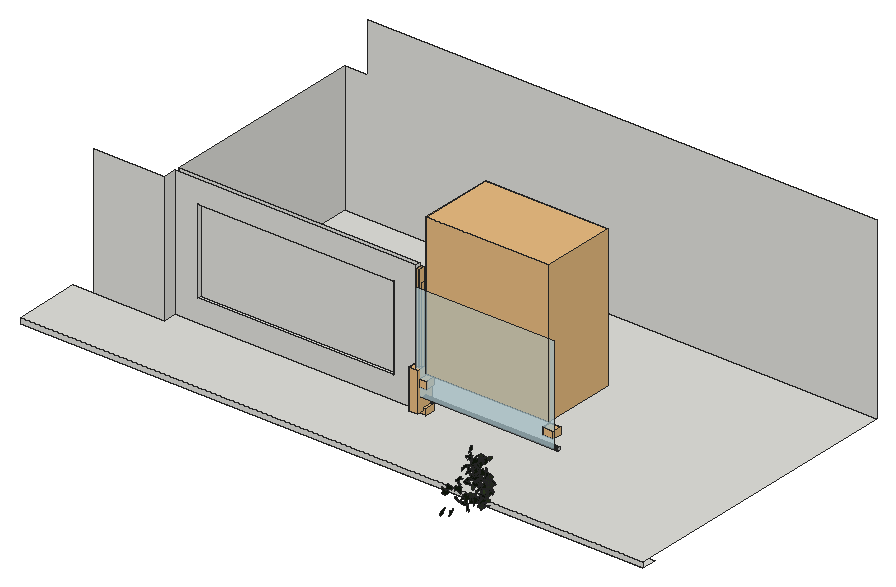
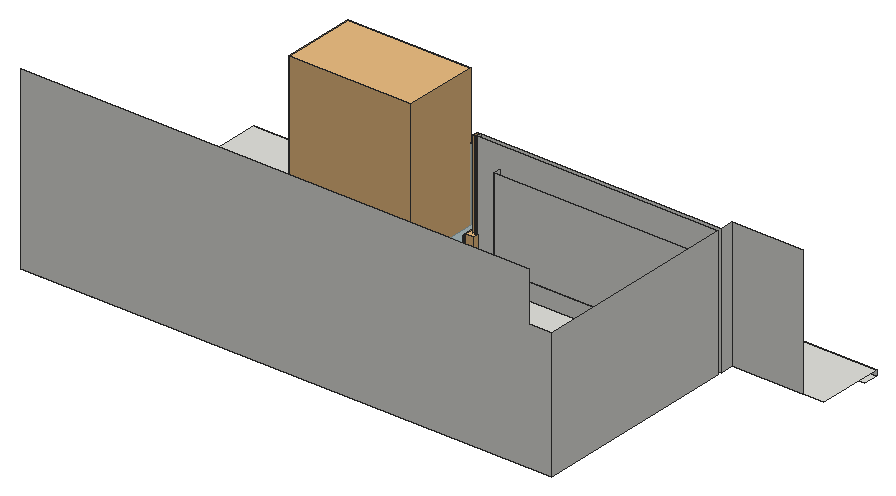
# SketchUp Ruby script. Lengths in inches.
U = 1.inch
M = Sketchup.active_model
def pt(a) = Geom::Point3d.new(a.map { |v| v * U })
def face(e, loops, mat)
  f = e.add_face(loops[0].map { |a| pt(a) })
  loops[1..].each { |l| e.add_face(l.map { |a| pt(a) }).erase! }
  f.material = f.back_material = mat if mat
  f
end
# faces: each face lists its corners as indices into pts; further lists are holes
def faces(e, pts, list, mat = nil) = list.each { |f| face(e, (f[0].is_a?(Array) ? f : [f]).map { |l| l.map { |i| pts[i] } }, mat) }
# xy, xz, yz: faces in a plane at the given z, y or x. An outline is a flat list of corners, or four numbers for a rectangle; further outlines are holes
def ring(l) = l.size == 4 ? [[l[0], l[1]], [l[2], l[1]], [l[2], l[3]], [l[0], l[3]]] : l.each_slice(2).to_a
def flat(e, list, mat, &to3) = list.each { |f| face(e, (f[0].is_a?(Array) ? f : [f]).map { |l| ring(l).map { |u, v| to3.(u, v) } }, mat) }
def xy(e, z, list, mat = nil) = flat(e, list, mat) { |x, y| [x, y, z] }
def xz(e, y, list, mat = nil) = flat(e, list, mat) { |x, z| [x, y, z] }
def yz(e, x, list, mat = nil) = flat(e, list, mat) { |y, z| [x, y, z] }
def lines(e, pts, list) = list.each { |a, b| e.add_line(pt(pts[a]), pt(pts[b])) }
# prism: a flat outline (further loops are holes) pulled along v
def prism(e, loops, v, mat = nil)
  f = face(e, loops, mat); d = Geom::Vector3d.new(v.map { |x| x * U })
  f.pushpull(f.normal.samedirection?(d) ? d.length : -d.length)
end
def box(e, o, s, mat = nil) = prism(e, [[o, [o[0] + s[0], o[1], o[2]], [o[0] + s[0], o[1] + s[1], o[2]], [o[0], o[1] + s[1], o[2]]]], [0, 0, s[2]], mat)
def at(x, y, z, deg = 0) = Geom::Transformation.translation(pt([x, y, z])) * Geom::Transformation.rotation(ORIGIN, Z_AXIS, deg.degrees)
def axes(o, x, y, z) = Geom::Transformation.new([*x, 0, *y, 0, *z, 0, *pt(o).to_a, 1])
def part(name) = M.definitions.add(name)
# library, detail: a bought-in or finely detailed component or shape, given as its bounding box
def library(name, o, s) = part(name).tap { |d| box(d.entities, o, s) }
def detail(e, o, s) = box(e.add_group.entities, o, s)
def put(e, d, t, mat = nil) = e.add_instance(d, t).tap { |i| i.material = mat if mat }
def group(e, t, mat = nil) = e.add_group.tap { |g| g.transformation = t; g.material = mat if mat }.entities
root = M.entities
M.materials.add("Glass Rail Metal").color = [192, 192, 192]
M.materials.add("[Translucent Glass Safety]").color = [204, 235, 244]
M.materials["[Translucent Glass Safety]"].alpha = 0.5
M.materials.add("[Translucent Glass Tinted]").color = [8, 201, 241]
M.materials["[Translucent Glass Tinted]"].alpha = 0.48
M.materials.add("efeu1").color = [18, 25, 13]
M.materials.add("efeu2").color = [43, 57, 29]
c1 = library("Group\#37",[0,0,0],[3.67,3.3,2.01])
c2 = library("Group\#43",[0,0,0],[50.8,6,878.92])
c3 = library("Group\#53",[0,0,0],[3.15,5.91,11.14])
c4 = library("Group\#15",[0.69,0,0.79],[0.62,1.89,30.3])
c5 = library("Group\#46",[0,0,0],[50.8,6,878.92])
c6 = library("glass bracket3",[-2.83,-0.98,-1],[3.67,3.29,2])
c7 = library("Palm+in+pot",[-44.1,-44.03,0.04],[106.77,95.72,88.04])
c8 = part("ivyleaf_9")
p = [[1.54,2.16,1.25],[1.36,2.04,1.19],[-0.21,0.99,0.68],[-0.71,1.11,0.82],[-0.85,0.86,0.67],[-0.8,0.17,0.21],
  [-0.9,-0.01,0.1],[-0.67,-0.16,-0.02],[-0.08,-0.08,-0.05],[-0.03,-0.6,-0.4],[0.65,-0.88,-0.66],[0.83,-0.6,-0.49],
  [1.29,-0.42,-0.43],[1.8125,-0.07,-0.26],[1.21,0.44,0.15]]
faces(c8.entities,p,[[0,1,2,3,4,5,6,7,8,9,10,11,12,13,14]],"efeu1")
c9 = part("ivyleaf_10")
p = [[0,0.5,-0.03],[-0.0625,2.02,-0.43],[-0.19,2.01,-0.46],[-0.54,1.05,-0.29],[-0.52,0.625,-0.18],[-0.83,0.76,-0.28],
  [-1.16,0.64,-0.33],[-1.15,0.33,-0.24],[-0.77,-0.39,0.02],[-0.3,-0.51,0.16],[0.04,-0.48,0.23],[-0.02,2.01,-0.4375],
  [-0.06,2.01,-0.43],[0.04,-0.49,0.23],[0.67,-0.49,0.14],[1.38,0.36,-0.2],[1.375,0.51,-0.24],[0.81,0.65,-0.19],
  [0.62,0.59,-0.15],[0.6,1.09,-0.28],[0.5,1.23,-0.31]]
faces(c9.entities,p,[[0,1,2,3,4,5,6,7,8,9,10],[11,12,0,13,14,15,16,17,18,19,20]],"efeu2")
c10 = library("glass bracket3\#1",[-0.84,-0.98,-1],[3.67,3.29,2])
prism(root,[[[415.35,181.67,254.4375],[415.35,181.84,254.35],[415.35,181.98,254.2],[415.35,182.09,254.02],[415.35,182.16,253.8125],[415.35,182.17,253.59],[415.35,182.14,253.375],[415.35,182.0625,253.18],[415.35,181.94,253.01],[415.35,181.79,252.88],[415.35,181.61,252.8],[415.35,181.43,252.78],[415.35,181.25,252.82],[415.35,181.08,252.91],[415.35,180.93,253.06],[415.35,180.83,253.24],[415.35,180.76,253.45],[415.35,180.75,253.67],[415.35,180.78,253.88],[415.35,180.86,254.09],[415.35,180.98,254.26],[415.35,181.13,254.38],[415.35,181.3,254.46],[415.35,181.49,254.48]]],[89.11,0,0],"Glass Rail Metal")
box(root,[415.02,177.2,254.7],[89.77,0.59,63.38],"[Translucent Glass Safety]")
xy(root,240.74,[[196.34,130,600,139.625]])
xy(root,244.35,[[196.34,130,600,130,600,319,255.63,319,255.63,184.12,411.76,184.12,411.76,181.4375,255.63,181.4375,255.63,172.6875,196.34,172.6875]])
xy(root,258.8125,[[270.09,181.4375,397.3,188.5625]])
xz(root,130,[[196.34,240.74,600,244.35]])
xz(root,172.6875,[[209.625,244.35,255.63,328.1875]])
xz(root,181.4375,[[[255.63,244.35,411.76,328.1875],[270.09,258.8125,397.3,313.73]]])
xz(root,184.12,[[255.63,244.35,411.76,328.1875]])
xz(root,188.5625,[[270.09,258.8125,397.3,313.73]])
xz(root,319,[[255.63,244.35,600,244.35,600,360,270.19,360,270.19,328.1875,255.63,328.1875]])
yz(root,255.63,[[172.6875,244.35,181.4375,328.1875],[184.12,244.35,319,328.1875]])
yz(root,270.09,[[181.4375,258.8125,188.5625,313.73]])
yz(root,397.3,[[181.4375,258.8125,188.5625,313.73]])
yz(root,411.76,[[181.4375,244.35,184.12,328.1875]])
put(root,c1,axes([408.92,179.59,243.35],[1.9,0,0],[0,1.9,0],[0,0,2.261]),"[Translucent Glass Tinted]")
put(root,c2,axes([413.71,179.56,248.78],[0,0.0748,0],[-0.0748,0,0.00001],[0.00001,0,0.08902]),"[Translucent Glass Tinted]")
put(root,c3,axes([411.3125,175.85,245.62],[1.9,0,0],[0,1.9,0],[0,0,2.261]),"[Translucent Glass Tinted]")
put(root,c4,axes([416.1,179.56,248.78],[0,1.9,0],[-1.9,0,0.00031],[0.00026,0,2.261]),"Glass Rail Metal")
put(root,c5,axes([415.35,179.56,248.78],[0,0.0748,0],[-0.0748,0,0.00001],[0.00001,0,0.08902]),"[Translucent Glass Tinted]")
put(root,c1,axes([419.68,179.59,247.89],[-1.9,0,0.00031],[0,1.9,0],[-0.00026,0,-2.261]),"[Translucent Glass Tinted]")
put(root,c6,axes([420.75,178.46,263.5625],[1.9,0,0],[0,1.9,0],[0,0,2.261]),"[Translucent Glass Tinted]")
put(root,c7,axes([454.51,199.21,269.81],[0.74365,0,0],[0,0.5,0],[0,0,1.0374]))
put(root,c8,axes([489.26,108.62,254.52],[0.59442,0.04762,1.18171],[-1.2151,0.20696,0.55776],[-0.17918,-1.24547,0.13787]))
put(root,c8,axes([489.92,123.09,263.95],[-0.23632,0.9466,-0.70763],[0.0907,-0.6777,-1.00862],[-1.25576,-0.22709,0.06031]))
put(root,c8,axes([489.8,104.18,244.44],[-0.48717,1.15827,0.44196],[0.13676,-0.40662,1.2924],[1.32543,0.46768,0.02909]))
put(root,c8,axes([490.71,109.53,258.73],[0.46963,0.40029,-1.13624],[-0.84856,-0.75927,-0.61453],[-0.92689,0.89792,-0.01311]))
put(root,c8,axes([491.32,124.37,256.75],[-0.12929,0.9505,-0.65584],[0.06165,-0.6283,-0.99615],[-1.23038,-0.13136,0.01901]))
put(root,c8,axes([492.43,109.09,243.9],[-0.46395,0.88248,0.8737],[-0.38333,0.7615,-1.02068],[-1.25881,-0.55714,-0.01119]))
put(root,c8,axes([492.08,114.92,260.75],[0.50243,0.7718,0.79926],[0.44241,0.65035,-0.93714],[-1.08994,0.61975,-0.01195]))
put(root,c8,axes([492.99,125.8125,244.46],[-1.16401,0.10836,-0.03835],[0.03948,-0.00498,-1.12655],[-0.11714,-1.07841,0.00135]))
put(root,c8,axes([492.79,122.28,264.03],[0.70443,-0.28766,-0.9331],[-0.88039,0.3749,-0.74133],[0.51027,1.04397,0.00911]))
put(root,c8,axes([492.25,114.53,256.4375],[-0.32312,-0.76804,-0.94362],[0.3738,0.83881,-0.85714],[1.22823,-0.45734,0.01261]))
put(root,c8,axes([491.68,114.18,249.6],[0.81283,-0.58166,0.82454],[0.66536,-0.49923,-0.98913],[0.82771,0.97252,-0.0146]))
put(root,c8,axes([492.22,114.51,259.49],[1.15165,-0.29641,-0.49126],[0.5136,-0.04902,1.14849],[-0.31455,-1.16525,0.07665]))
put(root,c8,axes([493.375,124.24,275.64],[-0.96606,0.3245,-0.62908],[0.60337,-0.23314,-0.98928],[-0.43074,-1.05435,0.02514]))
put(root,c8,axes([492.61,118.95,245.04],[1.18089,0.48616,0.00947],[-0.01579,0.01049,1.24438],[0.52491,-1.0934,0.01615]))
put(root,c9,axes([494.01,124.91,251.71],[-0.01496,0.96068,-0.5547],[-0.26695,0.51701,0.97515],[1.1563,0.13179,0.21795]))
put(root,c9,axes([493.64,126.24,247.0625],[1.13658,0.27915,-0.10532],[-0.09971,-0.04684,-1.13211],[-0.30482,1.05621,-0.02237]))
put(root,c8,axes([494.28,118.25,250.64],[-0.20997,0.14185,-1.19782],[0.28117,-1.1327,-0.19079],[-1.22134,-0.28515,0.162]))
put(root,c8,axes([495.04,124.27,259.86],[-1.22279,-0.30192,-0.02438],[0.0185,0.02674,-1.21845],[0.32653,-1.13214,-0.02227]))
put(root,c8,axes([495.25,125.76,256.46],[-0.91165,-0.17587,-0.62802],[0.65669,0.0302,-0.89312],[0.17367,-1.03743,0.08047]))
put(root,c8,axes([494.6,118.11,258.64],[1.3146,0.1766,0.29583],[0.30443,0.03824,-1.27916],[-0.19513,1.24943,-0.00266]))
put(root,c9,axes([495.26,126.13,264.75],[-0.70525,0.67366,0.48006],[0.35294,-0.32608,0.97571],[0.80827,0.73018,-0.00718]))
put(root,c9,axes([495.4,119.63,251.14],[-0.68522,-0.40785,-0.79658],[0.74981,0.33062,-0.78119],[0.56221,-0.93803,0.071]))
put(root,c8,axes([495.47,122.61,259.29],[-0.72287,0.34937,0.92842],[0.78728,-0.5216,0.78071],[0.67238,0.98634,0.08401]))
put(root,c8,axes([495.07,118.34,244.42],[0.19062,-0.19187,-1.17847],[1.23262,-0.10539,0.20344],[-0.14578,-1.14195,0.17923]))
put(root,c8,axes([496.06,118.46,265.13],[0.4824,1.15782,0.40717],[0.06927,0.39405,-1.28807],[-1.31818,0.44442,0.08131]))
put(root,c9,axes([495.97,125.23,249.87],[0.01531,0.00898,1.08629],[0.47437,-0.94782,0.00228],[1.02353,0.43915,-0.01731]))
put(root,c8,axes([495.92,127.1875,259.09],[0.26365,0.60698,-0.82966],[0.11096,0.80159,0.667],[1.0769,-0.2312,0.13439]))
put(root,c8,axes([496.58,124.47,257.15],[0.9974,-0.02515,-0.72931],[-0.74826,0.15106,-0.95456],[0.12013,1.14971,0.10946]))
put(root,c9,axes([496.63,126.25,246.34],[0.56465,-0.86551,0.1375],[-0.06856,0.11611,1.05159],[-0.9431,-0.52663,0.00587]))
put(root,c8,axes([496.37,118.125,273.8],[0.93319,0.76797,0.37537],[-0.29499,-0.23599,1.20225],[0.86766,-0.90619,0.00502]))
put(root,c8,axes([496.92,116.18,252.46],[-0.96397,-0.8,-0.3917],[0.33915,0.21348,-1.24554],[0.89271,-0.94496,0.05023]))
put(root,c8,axes([497.375,124.77,255.3],[0.82159,0.51454,-0.63696],[-0.55666,-0.33104,-0.95506],[-0.66066,0.91882,0.0126]))
put(root,c8,axes([497.67,122.72,264.42],[0.02039,-0.01486,1.25017],[-1.06964,-0.68164,0.00742],[0.73593,-0.99032,-0.02386]))
put(root,c8,axes([497.02,119.18,274.125],[0.02282,-0.38045,-1.09717],[0.76618,-0.81268,0.31957],[-0.93806,-0.67303,0.23433]))
put(root,c8,axes([496.93,120.54,271.07],[1.29376,0.42395,-0.07596],[-0.071,-0.03316,-1.32153],[-0.45915,1.1997,-0.00969]))
put(root,c8,axes([497.8125,127.9,268.34],[0.10158,0.85589,0.57328],[-0.02812,0.55542,-0.89227],[-1.09912,0.06489,0.07581]))
put(root,c9,axes([497.33,128.45,252.24],[-0.27962,0.6678,-0.68787],[0.16728,-0.64636,-0.74176],[-1.00123,-0.29449,0.06818]))
put(root,c8,axes([498.07,126.46,246.52],[-0.51845,-0.69757,0.72809],[0.42972,0.57602,0.88066],[-0.97703,0.62351,0.00099]))
put(root,c8,axes([497.29,128.67,250.08],[0.93369,0.14929,0.48545],[0.50216,0.04922,-0.91198],[-0.16725,0.98126,-0.02811]))
put(root,c8,axes([498.21,122.14,248.18],[-1.19875,-0.05103,-0.47341],[0.49073,0.02816,-1.15555],[0.06252,-1.19934,-0.00699]))
put(root,c8,axes([497.86,125.74,244.48],[0.03846,-0.01004,1.11078],[0.79742,0.77242,-0.01806],[-0.83354,0.73849,0.03398]))
put(root,c8,axes([498.91,124.87,260.09],[-0.57021,0.80716,0.39294],[-0.2596,0.29391,-1.00232],[-0.92684,-0.5789,0.039]))
put(root,c8,axes([499.3125,118.21,270.86],[-1.09828,0.58975,0.29064],[-0.27934,0.11083,-1.2221],[-0.6471,-1.04878,0.03428]))
put(root,c8,axes([499.33,122.64,271.09],[-0.48399,0.21608,-1.08328],[-0.9927,0.49034,0.51706],[0.57837,1.02243,-0.01903]))
put(root,c8,axes([497.89,128.9375,251.14],[0.73193,0.33999,-0.62217],[0.57673,0.26968,0.78854],[0.46868,-0.86282,0.0013]))
put(root,c8,axes([498.3,124.15,263.57],[-0.42369,-0.62657,-0.94047],[0.48431,0.78562,-0.76844],[1.08498,-0.59536,-0.02424]))
put(root,c8,axes([498.88,124.81,272.85],[0.73262,0.70684,-0.42724],[-0.33311,-0.27309,-1.01837],[-0.8177,0.74454,0.03207]))
put(root,c8,axes([499.125,121.33,266.38],[-1.17202,-0.47987,-0.06108],[0.0463,0.04824,-1.23372],[0.52007,-1.08572,-0.02782]))
put(root,c8,axes([499.16,123.875,259.02],[-1.06244,-0.31703,-0.00476],[0.00433,0.00247,-1.0749],[0.3424,-0.98375,-0.00117]))
put(root,c9,axes([499.01,128.86,262.73],[-0.5278,0.83865,0.21229],[-0.10608,0.17902,-1.00946],[-0.92613,-0.49845,-0.00536]))
put(root,c9,axes([499.9375,123.83,247.8],[-0.42018,-0.08789,0.95053],[-0.94622,-0.26144,-0.41401],[0.29668,-0.95831,0.02577]))
put(root,c8,axes([499.48,119.625,262.28],[0.32794,1.07427,-0.36795],[-0.15406,-0.32703,-1.16002],[-1.21176,0.33231,0.0479]))
put(root,c8,axes([498.92,125.71,242.52],[0.02375,0.19401,1.1371],[-0.13741,-1.08594,0.20306],[1.19138,-0.12911,0.00075]))
put(root,c9,axes([499.33,122.625,261.53],[-0.4946,-0.92051,-0.3972],[0.18685,0.34051,-1.06926],[1.05998,-0.48955,0.00314]))
put(root,c9,axes([499.84,124.1,269.86],[-0.58446,-0.67109,0.69207],[-0.41389,-0.54513,-0.89586],[0.93301,-0.66221,0.03612]))
put(root,c8,axes([499.29,121.08,266.4],[-0.48064,-1.03452,0.38549],[-0.10184,-0.36248,-1.1699],[1.18246,-0.45173,0.05593]))
put(root,c9,axes([500.11,124.25,244.1],[0.47919,0.04371,-1.01814],[-1.05788,0.05181,-0.45929],[0.03155,1.07358,0.06362]))
put(root,c8,axes([499.86,118.17,267.72],[0.00626,0.23484,1.24282],[-0.08344,1.19269,-0.24337],[-1.31265,-0.0747,0.0214]))
put(root,c9,axes([499.35,123.93,272.97],[-0.398,-0.79757,-0.68662],[0.33499,0.58356,-0.91322],[1.06685,-0.48078,0.0306]))
put(root,c8,axes([498.98,126.09,246.71],[-0.48769,-0.15086,-1.04299],[1.02077,0.33541,-0.49508],[0.3971,-1.04746,-0.00832]))
put(root,c9,axes([499.53,126.11,250.88],[1.01333,0.58244,-0.05122],[0.03833,0.0362,1.14845],[0.63011,-0.93886,0.01251]))
put(root,c8,axes([499.41,122.88,248.32],[0.06598,0.70876,0.74146],[-0.15711,-0.70051,0.73722],[1.0743,-0.14597,0.06228]))
put(root,c8,axes([500.07,120.97,262.73],[-0.9622,0.70983,-0.57843],[0.45503,-0.3636,-1.18451],[-0.86108,-0.98533,0.0204]))
put(root,c8,axes([500.28,126.12,243.96],[-0.38914,-0.21478,0.96345],[-0.8983,-0.40906,-0.43508],[0.49787,-0.90593,-0.03197]))
put(root,c8,axes([500.22,125.6875,252.71],[-0.50684,0.93397,-0.03433],[0.00924,-0.03264,-1.08703],[-1.00928,-0.46932,0.00729]))
put(root,c8,axes([499.02,123.09,259.01],[1.10397,-0.60906,-0.00991],[0.02094,0.05113,-1.23622],[0.65753,1.02096,0.056]))
put(root,c8,axes([500.1875,124.875,258.56],[-0.01206,0.79846,0.82459],[-0.12386,0.78798,-0.82695],[-1.20894,-0.0887,0.0765]))
put(root,c9,axes([500.125,128.3,250.86],[0.02132,-0.30179,0.95674],[-0.00056,-0.92014,-0.31392],[1.04563,0.00566,-0.01967]))
put(root,c8,axes([500.04,118.67,272.75],[0.56609,0.98108,0.66902],[0.26611,0.5968,-1.15538],[-1.23877,0.57653,0.05753]))
put(root,c8,axes([500.23,128.93,260.03],[0.49971,0.80893,-0.29277],[-0.12555,-0.25769,-0.96881],[-0.91647,0.47637,-0.02691]))
put(root,c8,axes([500.75,126.81,257.13],[-0.48232,0.83917,0.32159],[-0.20756,0.24751,-0.98722],[-0.94331,-0.48353,0.05279]))
put(root,c8,axes([499.3,126.25,242.76],[0.52702,0.09829,1.01098],[1.03188,0.17923,-0.51765],[-0.22067,1.07283,-0.00614]))
put(root,c8,axes([501.38,126.45,269.41],[-0.82945,0.04013,-0.74884],[-0.77635,-0.12684,0.79005],[-0.06237,1.04509,0.12464]))
put(root,c8,axes([500.28,121.49,270.95],[-0.18958,-1.21101,0.02323],[-0.03857,-0.01739,-1.27216],[1.30755,-0.17609,-0.03416]))
put(root,c8,axes([501.27,124.65,249.85],[-0.27198,0.87243,0.6464],[-0.40968,0.52447,-0.92548],[-1.08191,-0.41792,0.18795]))
put(root,c8,axes([501.07,117.61,275.22],[-0.57635,0.87058,-0.68833],[0.33657,-0.58486,-1.0614],[-1.13212,-0.61708,0.03488]))
put(root,c8,axes([501.03,126.3125,248.375],[-0.9583,0.20993,-0.28935],[0.28868,-0.03383,-0.98064],[-0.21084,-1.00046,-0.02756]))
put(root,c8,axes([500.9375,127.02,255.65],[-0.66578,0.36788,-0.7118],[0.45328,-0.5776,-0.71603],[-0.70624,-0.71752,0.21146]))
put(root,c8,axes([501.08,120.76,255.95],[-0.3237,0.56497,-0.99498],[-0.67377,0.73439,0.65429],[0.99295,0.6825,0.11961]))
put(root,c8,axes([501.29,117.6875,260.31],[0.54576,0.50327,-0.89773],[-0.68794,-0.58301,-0.74132],[-0.83142,0.81275,0.02411]))
put(root,c9,axes([501.41,131.22,253.28],[0.35995,-0.31545,-0.90782],[-0.6961,0.58282,-0.47852],[0.66265,0.7836,-0.00955]))
put(root,c8,axes([501.2,125.48,254.6875],[0.10401,0.06003,1.0835],[-0.07425,1.04434,-0.05597],[-1.12459,-0.0634,0.1039]))
put(root,c9,axes([500.79,127.21,248.11],[0.03446,-0.08816,1.00536],[-0.05047,0.96595,0.09322],[-1.04714,-0.04946,0.0286]))
put(root,c8,axes([501.24,124.47,248.56],[-1.03005,-0.52078,0.02857],[-0.02638,-0.0126,-1.13013],[0.5626,-0.95406,-0.00067]))
put(root,c10,axes([499.09,178.46,263.56],[1.9,0,0],[0,1.9,0],[0,0,2.261]),"[Translucent Glass Tinted]")
put(root,c8,axes([501.37,125.15,256.09],[-1.13655,0.01274,-0.23865],[0.24729,-0.03464,-1.09406],[-0.02141,-1.07653,0.03237]))
put(root,c9,axes([500.69,127.25,257.11],[-0.77746,-0.27748,-0.64093],[0.63721,0.18118,-0.80159],[0.35604,-0.93015,0.03506]))
put(root,c8,axes([501.29,130.17,250.45],[0.53262,0.59468,-0.53525],[-0.40638,-0.35502,-0.80162],[-0.74585,0.6181,0.05454]))
put(root,c9,axes([501.375,129.33,270.4],[-0.65522,-0.78029,0.09449],[-0.05988,-0.07198,-1.02793],[0.84629,-0.60922,0.00043]))
put(root,c9,axes([501.33,129.84,258.95],[-0.93089,-0.34626,-0.13785],[0.13002,0.05587,-0.96602],[0.37873,-0.87028,-0.00717]))
put(root,c8,axes([501.53,127.73,252.1],[0.20654,0.75058,0.61316],[0.0075,0.60018,-0.79699],[-1.03077,0.15476,0.11706]))
put(root,c9,axes([501.77,128.33,254.09],[-0.63065,-0.63198,0.5214],[-0.35182,-0.38533,-0.89259],[0.73992,-0.72187,0.01999]))
put(root,c8,axes([501.13,121.2,270.74],[-0.76076,-0.69143,-0.67415],[0.50181,0.452,-1.02652],[0.89214,-0.84384,0.00253]))
put(root,c9,axes([501.68,129.61,255.92],[-0.93614,0.36905,0.24353],[-0.28087,-0.05592,-0.99491],[-0.3415,-0.96568,0.15068]))
put(root,c8,axes([501.22,126.83,261.79],[-0.1569,0.18027,-1.0554],[0.77802,-0.71519,-0.23938],[-0.79611,-0.73447,-0.02594]))
put(root,c8,axes([501.58,123.82,264.49],[-0.579,-0.76276,0.58055],[-0.27648,-0.50061,-0.96709],[0.98267,-0.59028,0.06997]))
put(root,c8,axes([501.82,130.28,250.26],[-0.97571,-0.29641,0.05056],[-0.04796,-0.01608,-1.01974],[0.29684,-0.97689,0.00144]))
put(root,c8,axes([501.05,130.94,255.67],[1.01955,0.16715,-0.03853],[-0.03215,-0.04191,-1.03253],[-0.1685,1.01942,-0.03613]))
put(root,c8,axes([501.77,117.27,274.45],[-0.06336,0.27419,-1.32258],[0.25722,-1.24922,-0.29154],[-1.38126,-0.24521,0.00638]))
put(root,c8,axes([501.04,122.3,251.93],[1.272,0.22811,-0.04442],[-0.04665,-0.00157,-1.24763],[-0.24626,1.17855,0.00693]))
put(root,c9,axes([502.1,126.51,247.41],[-0.94678,-0.16942,0.53351],[-0.53669,-0.13074,-0.92808],[0.22891,-1.00726,0.03072]))
